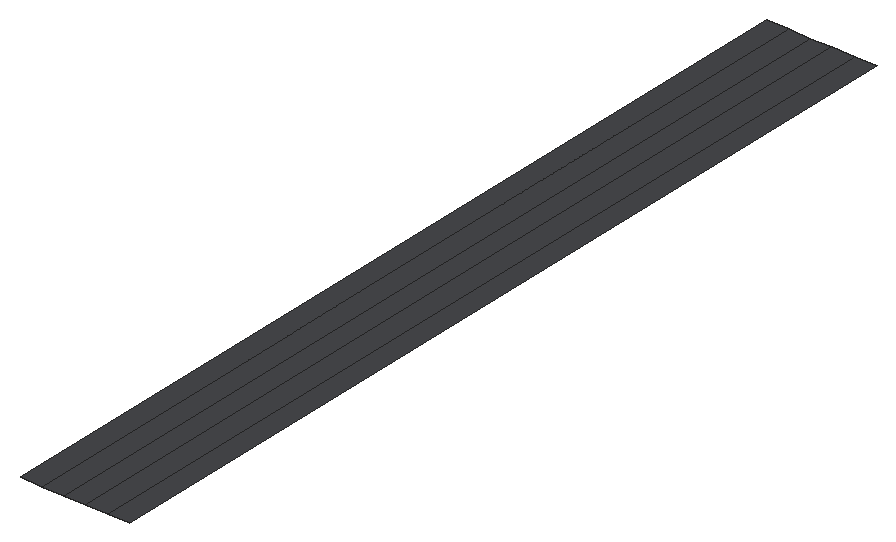
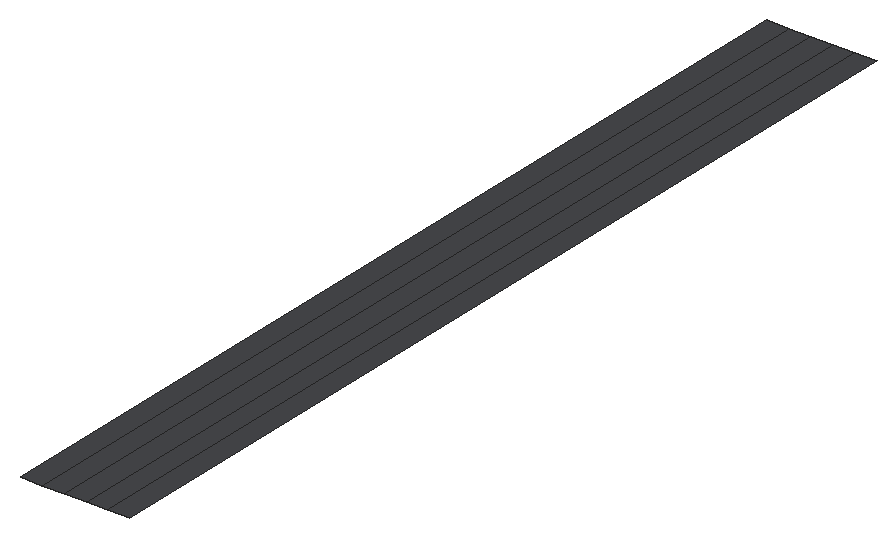
# SketchUp Ruby script. Lengths in inches.
U = 1.inch
M = Sketchup.active_model
def pt(a) = Geom::Point3d.new(a.map { |v| v * U })
def face(e, loops, mat)
  f = e.add_face(loops[0].map { |a| pt(a) })
  loops[1..].each { |l| e.add_face(l.map { |a| pt(a) }).erase! }
  f.material = f.back_material = mat if mat
  f
end
# faces: each face lists its corners as indices into pts; further lists are holes
def faces(e, pts, list, mat = nil) = list.each { |f| face(e, (f[0].is_a?(Array) ? f : [f]).map { |l| l.map { |i| pts[i] } }, mat) }
# xy, xz, yz: faces in a plane at the given z, y or x. An outline is a flat list of corners, or four numbers for a rectangle; further outlines are holes
def ring(l) = l.size == 4 ? [[l[0], l[1]], [l[2], l[1]], [l[2], l[3]], [l[0], l[3]]] : l.each_slice(2).to_a
def flat(e, list, mat, &to3) = list.each { |f| face(e, (f[0].is_a?(Array) ? f : [f]).map { |l| ring(l).map { |u, v| to3.(u, v) } }, mat) }
def xy(e, z, list, mat = nil) = flat(e, list, mat) { |x, y| [x, y, z] }
def xz(e, y, list, mat = nil) = flat(e, list, mat) { |x, z| [x, y, z] }
def yz(e, x, list, mat = nil) = flat(e, list, mat) { |y, z| [x, y, z] }
def lines(e, pts, list) = list.each { |a, b| e.add_line(pt(pts[a]), pt(pts[b])) }
# prism: a flat outline (further loops are holes) pulled along v
def prism(e, loops, v, mat = nil)
  f = face(e, loops, mat); d = Geom::Vector3d.new(v.map { |x| x * U })
  f.pushpull(f.normal.samedirection?(d) ? d.length : -d.length)
end
def box(e, o, s, mat = nil) = prism(e, [[o, [o[0] + s[0], o[1], o[2]], [o[0] + s[0], o[1] + s[1], o[2]], [o[0], o[1] + s[1], o[2]]]], [0, 0, s[2]], mat)
def at(x, y, z, deg = 0) = Geom::Transformation.translation(pt([x, y, z])) * Geom::Transformation.rotation(ORIGIN, Z_AXIS, deg.degrees)
def axes(o, x, y, z) = Geom::Transformation.new([*x, 0, *y, 0, *z, 0, *pt(o).to_a, 1])
def part(name) = M.definitions.add(name)
# library, detail: a bought-in or finely detailed component or shape, given as its bounding box
def library(name, o, s) = part(name).tap { |d| box(d.entities, o, s) }
def detail(e, o, s) = box(e.add_group.entities, o, s)
def put(e, d, t, mat = nil) = e.add_instance(d, t).tap { |i| i.material = mat if mat }
def group(e, t, mat = nil) = e.add_group.tap { |g| g.transformation = t; g.material = mat if mat }.entities
root = M.entities
M.materials.add("1432 AP 8245 TAR ROAD").color = [71, 72, 75]
xy(root,155.79,[[278.72,95.37,279,107.37]],"1432 AP 8245 TAR ROAD")
xy(root,155.8,[[278.15,95.37,278.43,107.37]],"1432 AP 8245 TAR ROAD")
p = [[277.59,107.37,155.82],[277.87,107.37,155.81],[277.87,95.37,155.81],[277.59,95.37,155.82],[278.15,107.37,155.8],[278.15,95.37,155.8],
  [278.43,107.37,155.8],[278.72,107.37,155.79],[278.72,95.37,155.79],[278.43,95.37,155.8]]
faces(root,p,[[0,1,2,3],[1,4,5,2],[6,7,8,9]],"1432 AP 8245 TAR ROAD")
